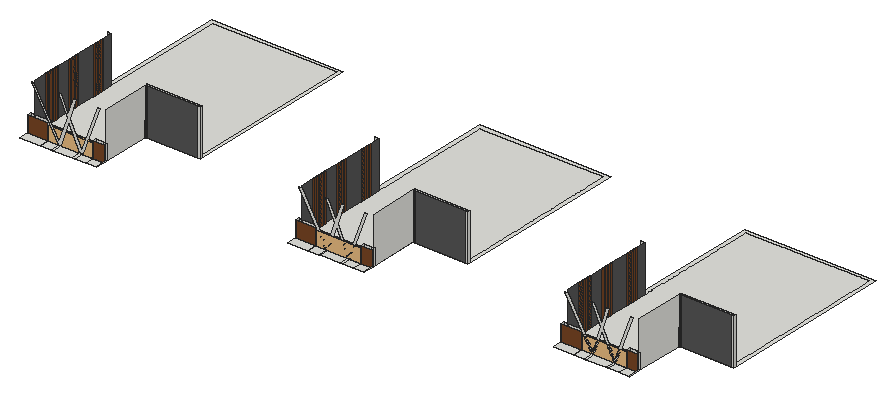
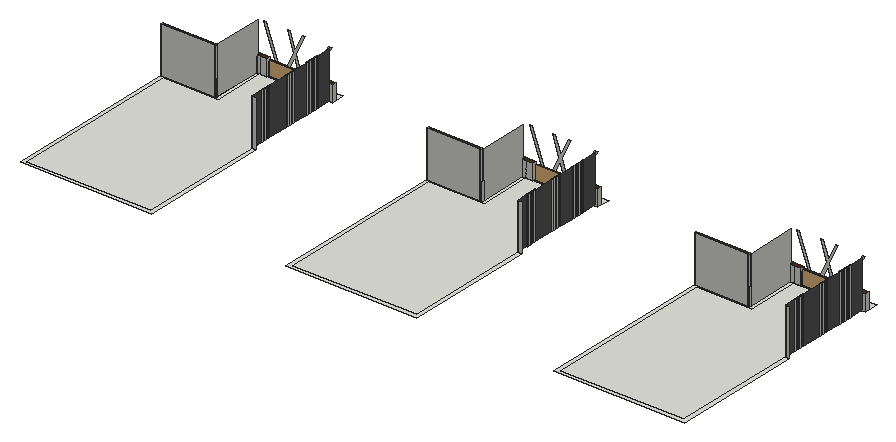
# SketchUp Ruby script. Lengths in inches.
U = 1.inch
M = Sketchup.active_model
def pt(a) = Geom::Point3d.new(a.map { |v| v * U })
def face(e, loops, mat)
  f = e.add_face(loops[0].map { |a| pt(a) })
  loops[1..].each { |l| e.add_face(l.map { |a| pt(a) }).erase! }
  f.material = f.back_material = mat if mat
  f
end
# faces: each face lists its corners as indices into pts; further lists are holes
def faces(e, pts, list, mat = nil) = list.each { |f| face(e, (f[0].is_a?(Array) ? f : [f]).map { |l| l.map { |i| pts[i] } }, mat) }
# xy, xz, yz: faces in a plane at the given z, y or x. An outline is a flat list of corners, or four numbers for a rectangle; further outlines are holes
def ring(l) = l.size == 4 ? [[l[0], l[1]], [l[2], l[1]], [l[2], l[3]], [l[0], l[3]]] : l.each_slice(2).to_a
def flat(e, list, mat, &to3) = list.each { |f| face(e, (f[0].is_a?(Array) ? f : [f]).map { |l| ring(l).map { |u, v| to3.(u, v) } }, mat) }
def xy(e, z, list, mat = nil) = flat(e, list, mat) { |x, y| [x, y, z] }
def xz(e, y, list, mat = nil) = flat(e, list, mat) { |x, z| [x, y, z] }
def yz(e, x, list, mat = nil) = flat(e, list, mat) { |y, z| [x, y, z] }
def lines(e, pts, list) = list.each { |a, b| e.add_line(pt(pts[a]), pt(pts[b])) }
# prism: a flat outline (further loops are holes) pulled along v
def prism(e, loops, v, mat = nil)
  f = face(e, loops, mat); d = Geom::Vector3d.new(v.map { |x| x * U })
  f.pushpull(f.normal.samedirection?(d) ? d.length : -d.length)
end
def box(e, o, s, mat = nil) = prism(e, [[o, [o[0] + s[0], o[1], o[2]], [o[0] + s[0], o[1] + s[1], o[2]], [o[0], o[1] + s[1], o[2]]]], [0, 0, s[2]], mat)
def at(x, y, z, deg = 0) = Geom::Transformation.translation(pt([x, y, z])) * Geom::Transformation.rotation(ORIGIN, Z_AXIS, deg.degrees)
def axes(o, x, y, z) = Geom::Transformation.new([*x, 0, *y, 0, *z, 0, *pt(o).to_a, 1])
def part(name) = M.definitions.add(name)
# library, detail: a bought-in or finely detailed component or shape, given as its bounding box
def library(name, o, s) = part(name).tap { |d| box(d.entities, o, s) }
def detail(e, o, s) = box(e.add_group.entities, o, s)
def put(e, d, t, mat = nil) = e.add_instance(d, t).tap { |i| i.material = mat if mat }
def group(e, t, mat = nil) = e.add_group.tap { |g| g.transformation = t; g.material = mat if mat }.entities
root = M.entities
M.materials.add("[Color M06]").color = [86, 86, 86]
M.materials.add("[Wood Veneer 01]").color = [120, 70, 37]
c1 = library("Glass Railing",[0,0,0],[139.5,4.76,42])
xy(root,399.3125,[[874.71,273.0625,933.87,301],[1661.09,273.0625,1720.25,301],[2441.46,273.0625,2500.62,301],[874.71,301,933.87,311.64],[1661.09,301,1720.25,311.64],
  [2441.46,301,2500.62,311.64]])
xy(root,399.625,[[933.87,273.0625,964.22,301],[964.22,273.0625,970.86,301],[970.86,273.0625,1028.09,301],[1028.09,273.0625,1035.11,301],[1035.11,273.0625,1066.62,301],
  [1066.62,273.0625,1098.03,301],[1720.25,273.0625,1750.6,301],[1750.6,273.0625,1757.23,301],[1757.23,273.0625,1814.46,301],[1814.46,273.0625,1821.48,301],
  [1821.48,273.0625,1852.99,301],[1852.99,273.0625,1884.4,301],[2500.62,273.0625,2530.97,301],[2530.97,273.0625,2537.61,301],[2537.61,273.0625,2594.84,301],
  [2594.84,273.0625,2601.86,301],[2601.86,273.0625,2633.37,301],[2633.37,273.0625,2664.78,301],[964.22,301,970.86,301,970.86,311.64,1028.09,311.64,1028.09,301,1035.11,301,1035.11,311.64,1087.38,311.64,1087.38,463.21,1249.94,463.21,1249.94,965.29,885.36,965.29,885.36,562.19,886.55,562.19,886.55,557.75,885.36,557.75,885.36,556.19,886.55,556.19,886.55,551.75,885.36,551.75,885.36,550.19,886.55,550.19,886.55,545.75,885.36,545.75,885.36,544.19,886.55,544.19,886.55,539.75,885.36,539.75,885.36,538.19,886.55,538.19,886.55,533.75,885.36,533.75,885.36,532.19,886.55,532.19,886.55,527.75,885.36,527.75,885.36,471.19,886.55,471.19,886.55,466.75,885.36,466.75,885.36,465.19,886.55,465.19,886.55,460.75,885.36,460.75,885.36,459.19,886.55,459.19,886.55,454.75,885.36,454.75,885.36,453.19,886.55,453.19,886.55,448.75,885.36,448.75,885.36,447.19,886.55,447.19,886.55,442.75,885.36,442.75,885.36,441.19,886.55,441.19,886.55,436.75,885.36,436.75,885.36,396.75,886.55,396.75,886.55,392.3125,885.36,392.3125,885.36,390.75,886.55,390.75,886.55,386.3125,885.36,386.3125,885.36,384.75,886.55,384.75,886.55,380.3125,885.36,380.3125,885.36,378.75,886.55,378.75,886.55,374.3125,885.36,374.3125,885.36,372.75,886.55,372.75,886.55,368.3125,885.36,368.3125,885.36,366.75,886.55,366.75,886.55,362.3125,885.36,362.3125,885.36,360.75,886.55,360.75,886.55,356.3125,885.36,356.3125,885.36,354.75,886.55,354.75,886.55,350.3125,885.36,350.3125,885.36,311.64,964.22,311.64],[933.87,301,964.22,311.64],
  [970.86,301,1028.09,311.64],[1035.11,301,1066.62,311.64],[1066.62,301,1098.03,311.64],[1750.6,301,1757.23,301,1757.23,311.64,1814.46,311.64,1814.46,301,1821.48,301,1821.48,311.64,1873.76,311.64,1873.76,463.21,2036.32,463.21,2036.32,965.29,1671.73,965.29,1671.73,562.19,1672.92,562.19,1672.92,557.75,1671.73,557.75,1671.73,556.19,1672.92,556.19,1672.92,551.75,1671.73,551.75,1671.73,550.19,1672.92,550.19,1672.92,545.75,1671.73,545.75,1671.73,544.19,1672.92,544.19,1672.92,539.75,1671.73,539.75,1671.73,538.19,1672.92,538.19,1672.92,533.75,1671.73,533.75,1671.73,532.19,1672.92,532.19,1672.92,527.75,1671.73,527.75,1671.73,471.19,1672.92,471.19,1672.92,466.75,1671.73,466.75,1671.73,465.19,1672.92,465.19,1672.92,460.75,1671.73,460.75,1671.73,459.19,1672.92,459.19,1672.92,454.75,1671.73,454.75,1671.73,453.19,1672.92,453.19,1672.92,448.75,1671.73,448.75,1671.73,447.19,1672.92,447.19,1672.92,442.75,1671.73,442.75,1671.73,441.19,1672.92,441.19,1672.92,436.75,1671.73,436.75,1671.73,396.75,1672.92,396.75,1672.92,392.3125,1671.73,392.3125,1671.73,390.75,1672.92,390.75,1672.92,386.3125,1671.73,386.3125,1671.73,384.75,1672.92,384.75,1672.92,380.3125,1671.73,380.3125,1671.73,378.75,1672.92,378.75,1672.92,374.3125,1671.73,374.3125,1671.73,372.75,1672.92,372.75,1672.92,368.3125,1671.73,368.3125,1671.73,366.75,1672.92,366.75,1672.92,362.3125,1671.73,362.3125,1671.73,360.75,1672.92,360.75,1672.92,356.3125,1671.73,356.3125,1671.73,354.75,1672.92,354.75,1672.92,350.3125,1671.73,350.3125,1671.73,311.64,1750.6,311.64],[1720.25,301,1750.6,311.64],
  [1757.23,301,1814.46,311.64],[1821.48,301,1852.99,311.64],[1852.99,301,1884.4,311.64],[2530.97,301,2537.61,301,2537.61,311.64,2594.84,311.64,2594.84,301,2601.86,301,2601.86,311.64,2654.13,311.64,2654.13,463.21,2816.69,463.21,2816.69,965.29,2452.11,965.29,2452.11,562.19,2453.3,562.19,2453.3,557.75,2452.11,557.75,2452.11,556.19,2453.3,556.19,2453.3,551.75,2452.11,551.75,2452.11,550.19,2453.3,550.19,2453.3,545.75,2452.11,545.75,2452.11,544.19,2453.3,544.19,2453.3,539.75,2452.11,539.75,2452.11,538.19,2453.3,538.19,2453.3,533.75,2452.11,533.75,2452.11,532.19,2453.3,532.19,2453.3,527.75,2452.11,527.75,2452.11,471.19,2453.3,471.19,2453.3,466.75,2452.11,466.75,2452.11,465.19,2453.3,465.19,2453.3,460.75,2452.11,460.75,2452.11,459.19,2453.3,459.19,2453.3,454.75,2452.11,454.75,2452.11,453.19,2453.3,453.19,2453.3,448.75,2452.11,448.75,2452.11,447.19,2453.3,447.19,2453.3,442.75,2452.11,442.75,2452.11,441.19,2453.3,441.19,2453.3,436.75,2452.11,436.75,2452.11,396.75,2453.3,396.75,2453.3,392.3125,2452.11,392.3125,2452.11,390.75,2453.3,390.75,2453.3,386.3125,2452.11,386.3125,2452.11,384.75,2453.3,384.75,2453.3,380.3125,2452.11,380.3125,2452.11,378.75,2453.3,378.75,2453.3,374.3125,2452.11,374.3125,2452.11,372.75,2453.3,372.75,2453.3,368.3125,2452.11,368.3125,2452.11,366.75,2453.3,366.75,2453.3,362.3125,2452.11,362.3125,2452.11,360.75,2453.3,360.75,2453.3,356.3125,2452.11,356.3125,2452.11,354.75,2453.3,354.75,2453.3,350.3125,2452.11,350.3125,2452.11,311.64,2530.97,311.64],[2500.62,301,2530.97,311.64],
  [2537.61,301,2594.84,311.64],[2601.86,301,2633.37,311.64],[2633.37,301,2664.78,311.64],[1087.38,311.64,1098.03,311.64,1098.03,459.0625,1260.59,459.0625,1260.59,975.9375,874.71,975.9375,874.71,593.65,885.36,593.65,885.36,965.29,1249.94,965.29,1249.94,463.21,1087.38,463.21],[1873.76,311.64,1884.4,311.64,1884.4,459.0625,2046.96,459.0625,2046.96,975.9375,1661.09,975.9375,1661.09,593.65,1671.73,593.65,1671.73,965.29,2036.32,965.29,2036.32,463.21,1873.76,463.21],
  [2654.13,311.64,2664.78,311.64,2664.78,459.0625,2827.34,459.0625,2827.34,975.9375,2441.46,975.9375,2441.46,593.65,2452.11,593.65,2452.11,965.29,2816.69,965.29,2816.69,463.21,2654.13,463.21],[1098.03,452.5625,1103.7,459.0625],[1103.7,452.5625,1260.59,459.0625],[1884.4,452.5625,1890.08,459.0625],[1890.08,452.5625,2046.96,459.0625],
  [2664.78,452.5625,2670.45,459.0625],[2670.45,452.5625,2827.34,459.0625]])
xz(root,301,[[964.22,399.625,970.86,399.625,994.52,471.53,1028.09,399.625,1035.11,399.625,1084.99,536.4375,1078.92,536.4375,1031.69,406.9,997.33,480.06,1015.88,536.4375,1009.09,536.4375,993.37,488.5,970.86,536.4375,964.22,536.4375,990.58,479.98,966.65,407.03,893.1875,536.4375,885.36,536.4375],[1750.6,399.625,1757.23,399.625,1780.9,471.53,1814.46,399.625,1821.48,399.625,1871.36,536.4375,1865.29,536.4375,1818.07,406.9,1783.71,480.06,1802.26,536.4375,1795.47,536.4375,1779.75,488.5,1757.23,536.4375,1750.6,536.4375,1776.95,479.98,1753.03,407.03,1679.5625,536.4375,1671.73,536.4375],[2530.97,399.625,2537.61,399.625,2561.27,471.53,2594.84,399.625,2601.86,399.625,2651.74,536.4375,2645.67,536.4375,2598.44,406.9,2564.08,480.06,2582.63,536.4375,2575.84,536.4375,2560.12,488.5,2537.61,536.4375,2530.97,536.4375,2557.33,479.98,2533.4,407.03,2459.9375,536.4375,2452.11,536.4375]])
xz(root,301,[[874.71,399.3125,933.87,446.625],[1661.09,399.3125,1720.25,446.625],[2441.46,399.3125,2500.62,446.625],[1066.62,399.625,1098.03,446.625],[1852.99,399.625,1884.4,446.625],
  [2633.37,399.625,2664.78,446.625]],"[Wood Veneer 01]")
xz(root,311.64,[[874.71,399.3125,885.36,446.625],[885.36,399.3125,933.87,399.625],[1661.09,399.3125,1671.73,446.625],[1671.73,399.3125,1720.25,399.625],[2441.46,399.3125,2452.11,446.625],
  [2452.11,399.3125,2500.62,399.625],[885.36,399.625,933.87,446.625],[1066.62,399.625,1087.38,446.625],[1087.38,399.625,1098.03,446.625],[1671.73,399.625,1720.25,446.625],
  [1852.99,399.625,1873.76,446.625],[1873.76,399.625,1884.4,446.625],[2452.11,399.625,2500.62,446.625],[2633.37,399.625,2654.13,446.625],[2654.13,399.625,2664.78,446.625]])
xz(root,350.3125,[[885.36,399.625,886.55,536.4375],[1671.73,399.625,1672.92,536.4375],[2452.11,399.625,2453.3,536.4375]],"[Wood Veneer 01]")
xz(root,354.75,[[885.36,399.625,886.55,536.4375],[1671.73,399.625,1672.92,536.4375],[2452.11,399.625,2453.3,536.4375]])
xz(root,356.3125,[[885.36,399.625,886.55,536.4375],[1671.73,399.625,1672.92,536.4375],[2452.11,399.625,2453.3,536.4375]],"[Wood Veneer 01]")
xz(root,360.75,[[885.36,399.625,886.55,536.4375],[1671.73,399.625,1672.92,536.4375],[2452.11,399.625,2453.3,536.4375]])
xz(root,362.3125,[[885.36,399.625,886.55,536.4375],[1671.73,399.625,1672.92,536.4375],[2452.11,399.625,2453.3,536.4375]],"[Wood Veneer 01]")
xz(root,366.75,[[885.36,399.625,886.55,536.4375],[1671.73,399.625,1672.92,536.4375],[2452.11,399.625,2453.3,536.4375]])
xz(root,368.3125,[[885.36,399.625,886.55,536.4375],[1671.73,399.625,1672.92,536.4375],[2452.11,399.625,2453.3,536.4375]],"[Wood Veneer 01]")
xz(root,372.75,[[885.36,399.625,886.55,536.4375],[1671.73,399.625,1672.92,536.4375],[2452.11,399.625,2453.3,536.4375]])
xz(root,374.3125,[[885.36,399.625,886.55,536.4375],[1671.73,399.625,1672.92,536.4375],[2452.11,399.625,2453.3,536.4375]],"[Wood Veneer 01]")
xz(root,378.75,[[885.36,399.625,886.55,536.4375],[1671.73,399.625,1672.92,536.4375],[2452.11,399.625,2453.3,536.4375]])
xz(root,380.3125,[[885.36,399.625,886.55,536.4375],[1671.73,399.625,1672.92,536.4375],[2452.11,399.625,2453.3,536.4375]],"[Wood Veneer 01]")
xz(root,384.75,[[885.36,399.625,886.55,536.4375],[1671.73,399.625,1672.92,536.4375],[2452.11,399.625,2453.3,536.4375]])
xz(root,386.3125,[[885.36,399.625,886.55,536.4375],[1671.73,399.625,1672.92,536.4375],[2452.11,399.625,2453.3,536.4375]],"[Wood Veneer 01]")
xz(root,390.75,[[885.36,399.625,886.55,536.4375],[1671.73,399.625,1672.92,536.4375],[2452.11,399.625,2453.3,536.4375]])
xz(root,392.3125,[[885.36,399.625,886.55,536.4375],[1671.73,399.625,1672.92,536.4375],[2452.11,399.625,2453.3,536.4375]],"[Wood Veneer 01]")
xz(root,396.75,[[885.36,399.625,886.55,536.4375],[1671.73,399.625,1672.92,536.4375],[2452.11,399.625,2453.3,536.4375]])
xz(root,436.75,[[885.36,399.625,886.55,536.4375],[1671.73,399.625,1672.92,536.4375],[2452.11,399.625,2453.3,536.4375]],"[Wood Veneer 01]")
xz(root,441.19,[[885.36,399.625,886.55,536.4375],[1671.73,399.625,1672.92,536.4375],[2452.11,399.625,2453.3,536.4375]])
xz(root,442.75,[[885.36,399.625,886.55,536.4375],[1671.73,399.625,1672.92,536.4375],[2452.11,399.625,2453.3,536.4375]],"[Wood Veneer 01]")
xz(root,447.19,[[885.36,399.625,886.55,536.4375],[1671.73,399.625,1672.92,536.4375],[2452.11,399.625,2453.3,536.4375]])
xz(root,448.75,[[885.36,399.625,886.55,536.4375],[1671.73,399.625,1672.92,536.4375],[2452.11,399.625,2453.3,536.4375]],"[Wood Veneer 01]")
xz(root,452.5625,[[1098.03,399.625,1103.7,536.4375],[1253.34,399.625,1260.59,536.4375],[1884.4,399.625,1890.08,536.4375],[2039.72,399.625,2046.96,536.4375],[2664.78,399.625,2670.45,536.4375],
  [2820.09,399.625,2827.34,536.4375]])
xz(root,452.5625,[[1103.7,399.625,1253.34,536.4375],[1890.08,399.625,2039.72,536.4375],[2670.45,399.625,2820.09,536.4375]],"[Color M06]")
xz(root,453.19,[[885.36,399.625,886.55,536.4375],[1671.73,399.625,1672.92,536.4375],[2452.11,399.625,2453.3,536.4375]])
xz(root,454.75,[[885.36,399.625,886.55,536.4375],[1671.73,399.625,1672.92,536.4375],[2452.11,399.625,2453.3,536.4375]],"[Wood Veneer 01]")
xz(root,459.0625,[[1098.03,399.625,1103.7,536.4375],[1103.7,399.625,1260.59,536.4375],[1884.4,399.625,1890.08,536.4375],[1890.08,399.625,2046.96,536.4375],[2664.78,399.625,2670.45,536.4375],
  [2670.45,399.625,2827.34,536.4375]])
xz(root,459.19,[[885.36,399.625,886.55,536.4375],[1671.73,399.625,1672.92,536.4375],[2452.11,399.625,2453.3,536.4375]])
xz(root,460.75,[[885.36,399.625,886.55,536.4375],[1671.73,399.625,1672.92,536.4375],[2452.11,399.625,2453.3,536.4375]],"[Wood Veneer 01]")
xz(root,465.19,[[885.36,399.625,886.55,536.4375],[1671.73,399.625,1672.92,536.4375],[2452.11,399.625,2453.3,536.4375]])
xz(root,466.75,[[885.36,399.625,886.55,536.4375],[1671.73,399.625,1672.92,536.4375],[2452.11,399.625,2453.3,536.4375]],"[Wood Veneer 01]")
xz(root,471.19,[[885.36,399.625,886.55,536.4375],[1671.73,399.625,1672.92,536.4375],[2452.11,399.625,2453.3,536.4375]])
xz(root,527.75,[[885.36,399.625,886.55,536.4375],[1671.73,399.625,1672.92,536.4375],[2452.11,399.625,2453.3,536.4375]],"[Wood Veneer 01]")
xz(root,532.19,[[885.36,399.625,886.55,536.4375],[1671.73,399.625,1672.92,536.4375],[2452.11,399.625,2453.3,536.4375]])
xz(root,533.75,[[885.36,399.625,886.55,536.4375],[1671.73,399.625,1672.92,536.4375],[2452.11,399.625,2453.3,536.4375]],"[Wood Veneer 01]")
xz(root,538.19,[[885.36,399.625,886.55,536.4375],[1671.73,399.625,1672.92,536.4375],[2452.11,399.625,2453.3,536.4375]])
xz(root,539.75,[[885.36,399.625,886.55,536.4375],[1671.73,399.625,1672.92,536.4375],[2452.11,399.625,2453.3,536.4375]],"[Wood Veneer 01]")
xz(root,544.19,[[885.36,399.625,886.55,536.4375],[1671.73,399.625,1672.92,536.4375],[2452.11,399.625,2453.3,536.4375]])
xz(root,545.75,[[885.36,399.625,886.55,536.4375],[1671.73,399.625,1672.92,536.4375],[2452.11,399.625,2453.3,536.4375]],"[Wood Veneer 01]")
xz(root,550.19,[[885.36,399.625,886.55,536.4375],[1671.73,399.625,1672.92,536.4375],[2452.11,399.625,2453.3,536.4375]])
xz(root,551.75,[[885.36,399.625,886.55,536.4375],[1671.73,399.625,1672.92,536.4375],[2452.11,399.625,2453.3,536.4375]],"[Wood Veneer 01]")
xz(root,556.19,[[885.36,399.625,886.55,536.4375],[1671.73,399.625,1672.92,536.4375],[2452.11,399.625,2453.3,536.4375]])
xz(root,557.75,[[885.36,399.625,886.55,536.4375],[1671.73,399.625,1672.92,536.4375],[2452.11,399.625,2453.3,536.4375]],"[Wood Veneer 01]")
xz(root,562.19,[[885.36,399.625,886.55,536.4375],[1671.73,399.625,1672.92,536.4375],[2452.11,399.625,2453.3,536.4375]])
xz(root,593.65,[[874.71,399.625,885.36,536.4375],[1661.09,399.625,1671.73,536.4375],[2441.46,399.625,2452.11,536.4375]])
yz(root,874.71,[[301,399.3125,311.64,446.625]])
yz(root,885.36,[[354.75,399.625,356.3125,536.4375],[360.75,399.625,362.3125,536.4375],[366.75,399.625,368.3125,536.4375],[372.75,399.625,374.3125,536.4375],[378.75,399.625,380.3125,536.4375],
  [384.75,399.625,386.3125,536.4375],[390.75,399.625,392.3125,536.4375],[441.19,399.625,442.75,536.4375],[447.19,399.625,448.75,536.4375],[453.19,399.625,454.75,536.4375],
  [459.19,399.625,460.75,536.4375],[465.19,399.625,466.75,536.4375],[532.19,399.625,533.75,536.4375],[538.19,399.625,539.75,536.4375],[544.19,399.625,545.75,536.4375],
  [550.19,399.625,551.75,536.4375],[556.19,399.625,557.75,536.4375]])
yz(root,885.36,[[311.64,399.625,350.3125,536.4375],[396.75,399.625,436.75,536.4375],[471.19,399.625,527.75,536.4375],[562.19,399.625,593.65,536.4375]],"[Color M06]")
yz(root,886.55,[[350.3125,399.625,354.75,536.4375],[356.3125,399.625,360.75,536.4375],[362.3125,399.625,366.75,536.4375],[368.3125,399.625,372.75,536.4375],[374.3125,399.625,378.75,536.4375],
  [380.3125,399.625,384.75,536.4375],[386.3125,399.625,390.75,536.4375],[392.3125,399.625,396.75,536.4375],[436.75,399.625,441.19,536.4375],[442.75,399.625,447.19,536.4375],
  [448.75,399.625,453.19,536.4375],[454.75,399.625,459.19,536.4375],[460.75,399.625,465.19,536.4375],[466.75,399.625,471.19,536.4375],[527.75,399.625,532.19,536.4375],
  [533.75,399.625,538.19,536.4375],[539.75,399.625,544.19,536.4375],[545.75,399.625,550.19,536.4375],[551.75,399.625,556.19,536.4375],[557.75,399.625,562.19,536.4375]],"[Wood Veneer 01]")
yz(root,933.87,[[273.0625,399.3125,301,399.625],[301,399.3125,311.64,399.625],[301,399.625,311.64,446.625]])
yz(root,1066.62,[[301,399.625,311.64,446.625]])
yz(root,1098.03,[[273.0625,399.625,301,400.68],[301,399.625,308.24,400.68],[308.24,399.625,311.64,446.625],[311.64,399.625,311.64,449.125,308.24,449.125,308.24,536.4375,452.5625,536.4375,452.5625,399.625],[452.5625,399.625,459.0625,451.1875]])
yz(root,1103.7,[[452.5625,399.625,459.0625,536.4375]])
yz(root,1260.59,[[452.5625,399.625,459.0625,536.4375]])
yz(root,1661.09,[[301,399.3125,311.64,446.625]])
yz(root,1671.73,[[354.75,399.625,356.3125,536.4375],[360.75,399.625,362.3125,536.4375],[366.75,399.625,368.3125,536.4375],[372.75,399.625,374.3125,536.4375],[378.75,399.625,380.3125,536.4375],
  [384.75,399.625,386.3125,536.4375],[390.75,399.625,392.3125,536.4375],[441.19,399.625,442.75,536.4375],[447.19,399.625,448.75,536.4375],[453.19,399.625,454.75,536.4375],
  [459.19,399.625,460.75,536.4375],[465.19,399.625,466.75,536.4375],[532.19,399.625,533.75,536.4375],[538.19,399.625,539.75,536.4375],[544.19,399.625,545.75,536.4375],
  [550.19,399.625,551.75,536.4375],[556.19,399.625,557.75,536.4375]])
yz(root,1671.73,[[311.64,399.625,350.3125,536.4375],[396.75,399.625,436.75,536.4375],[471.19,399.625,527.75,536.4375],[562.19,399.625,593.65,536.4375]],"[Color M06]")
yz(root,1672.92,[[350.3125,399.625,354.75,536.4375],[356.3125,399.625,360.75,536.4375],[362.3125,399.625,366.75,536.4375],[368.3125,399.625,372.75,536.4375],[374.3125,399.625,378.75,536.4375],
  [380.3125,399.625,384.75,536.4375],[386.3125,399.625,390.75,536.4375],[392.3125,399.625,396.75,536.4375],[436.75,399.625,441.19,536.4375],[442.75,399.625,447.19,536.4375],
  [448.75,399.625,453.19,536.4375],[454.75,399.625,459.19,536.4375],[460.75,399.625,465.19,536.4375],[466.75,399.625,471.19,536.4375],[527.75,399.625,532.19,536.4375],
  [533.75,399.625,538.19,536.4375],[539.75,399.625,544.19,536.4375],[545.75,399.625,550.19,536.4375],[551.75,399.625,556.19,536.4375],[557.75,399.625,562.19,536.4375]],"[Wood Veneer 01]")
yz(root,1720.25,[[273.0625,399.3125,301,399.625],[301,399.3125,311.64,399.625],[301,399.625,311.64,446.625]])
yz(root,1852.99,[[301,399.625,311.64,446.625]])
yz(root,1884.4,[[273.0625,399.625,301,400.68],[301,399.625,308.24,400.68],[308.24,399.625,311.64,446.625],[311.64,399.625,311.64,449.125,308.24,449.125,308.24,536.4375,452.5625,536.4375,452.5625,399.625],[452.5625,399.625,459.0625,451.1875]])
yz(root,1890.08,[[452.5625,399.625,459.0625,536.4375]])
yz(root,2046.96,[[452.5625,399.625,459.0625,536.4375]])
yz(root,2441.46,[[301,399.3125,311.64,446.625]])
yz(root,2452.11,[[354.75,399.625,356.3125,536.4375],[360.75,399.625,362.3125,536.4375],[366.75,399.625,368.3125,536.4375],[372.75,399.625,374.3125,536.4375],[378.75,399.625,380.3125,536.4375],
  [384.75,399.625,386.3125,536.4375],[390.75,399.625,392.3125,536.4375],[441.19,399.625,442.75,536.4375],[447.19,399.625,448.75,536.4375],[453.19,399.625,454.75,536.4375],
  [459.19,399.625,460.75,536.4375],[465.19,399.625,466.75,536.4375],[532.19,399.625,533.75,536.4375],[538.19,399.625,539.75,536.4375],[544.19,399.625,545.75,536.4375],
  [550.19,399.625,551.75,536.4375],[556.19,399.625,557.75,536.4375]])
yz(root,2452.11,[[311.64,399.625,350.3125,536.4375],[396.75,399.625,436.75,536.4375],[471.19,399.625,527.75,536.4375],[562.19,399.625,593.65,536.4375]],"[Color M06]")
yz(root,2453.3,[[350.3125,399.625,354.75,536.4375],[356.3125,399.625,360.75,536.4375],[362.3125,399.625,366.75,536.4375],[368.3125,399.625,372.75,536.4375],[374.3125,399.625,378.75,536.4375],
  [380.3125,399.625,384.75,536.4375],[386.3125,399.625,390.75,536.4375],[392.3125,399.625,396.75,536.4375],[436.75,399.625,441.19,536.4375],[442.75,399.625,447.19,536.4375],
  [448.75,399.625,453.19,536.4375],[454.75,399.625,459.19,536.4375],[460.75,399.625,465.19,536.4375],[466.75,399.625,471.19,536.4375],[527.75,399.625,532.19,536.4375],
  [533.75,399.625,538.19,536.4375],[539.75,399.625,544.19,536.4375],[545.75,399.625,550.19,536.4375],[551.75,399.625,556.19,536.4375],[557.75,399.625,562.19,536.4375]],"[Wood Veneer 01]")
yz(root,2500.62,[[273.0625,399.3125,301,399.625],[301,399.3125,311.64,399.625],[301,399.625,311.64,446.625]])
yz(root,2633.37,[[301,399.625,311.64,446.625]])
yz(root,2664.78,[[273.0625,399.625,301,400.68],[301,399.625,308.24,400.68],[308.24,399.625,311.64,446.625],[311.64,399.625,311.64,449.125,308.24,449.125,308.24,536.4375,452.5625,536.4375,452.5625,399.625],[452.5625,399.625,459.0625,451.1875]])
yz(root,2670.45,[[452.5625,399.625,459.0625,536.4375]])
yz(root,2827.34,[[452.5625,399.625,459.0625,536.4375]])
put(root,c1,axes([1720.25,301,399.625],[0.95159,0,0],[0,1,0],[0,0,1]))
put(root,c1,axes([933.87,301,399.625],[0.95159,0,0],[0,1,0],[0,0,1]))
put(root,c1,axes([2500.62,301,399.625],[0.95159,0,0],[0,1,0],[0,0,1]))
